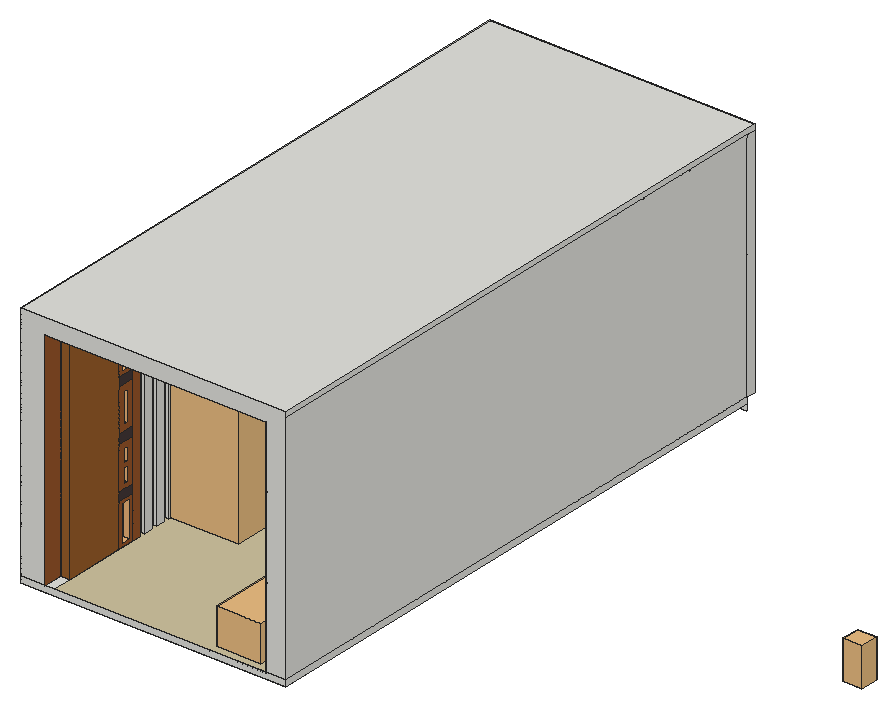
# SketchUp Ruby script. Lengths in inches.
U = 1.inch
M = Sketchup.active_model
def pt(a) = Geom::Point3d.new(a.map { |v| v * U })
def face(e, loops, mat)
  f = e.add_face(loops[0].map { |a| pt(a) })
  loops[1..].each { |l| e.add_face(l.map { |a| pt(a) }).erase! }
  f.material = f.back_material = mat if mat
  f
end
# faces: each face lists its corners as indices into pts; further lists are holes
def faces(e, pts, list, mat = nil) = list.each { |f| face(e, (f[0].is_a?(Array) ? f : [f]).map { |l| l.map { |i| pts[i] } }, mat) }
# xy, xz, yz: faces in a plane at the given z, y or x. An outline is a flat list of corners, or four numbers for a rectangle; further outlines are holes
def ring(l) = l.size == 4 ? [[l[0], l[1]], [l[2], l[1]], [l[2], l[3]], [l[0], l[3]]] : l.each_slice(2).to_a
def flat(e, list, mat, &to3) = list.each { |f| face(e, (f[0].is_a?(Array) ? f : [f]).map { |l| ring(l).map { |u, v| to3.(u, v) } }, mat) }
def xy(e, z, list, mat = nil) = flat(e, list, mat) { |x, y| [x, y, z] }
def xz(e, y, list, mat = nil) = flat(e, list, mat) { |x, z| [x, y, z] }
def yz(e, x, list, mat = nil) = flat(e, list, mat) { |y, z| [x, y, z] }
def lines(e, pts, list) = list.each { |a, b| e.add_line(pt(pts[a]), pt(pts[b])) }
# prism: a flat outline (further loops are holes) pulled along v
def prism(e, loops, v, mat = nil)
  f = face(e, loops, mat); d = Geom::Vector3d.new(v.map { |x| x * U })
  f.pushpull(f.normal.samedirection?(d) ? d.length : -d.length)
end
def box(e, o, s, mat = nil) = prism(e, [[o, [o[0] + s[0], o[1], o[2]], [o[0] + s[0], o[1] + s[1], o[2]], [o[0], o[1] + s[1], o[2]]]], [0, 0, s[2]], mat)
def at(x, y, z, deg = 0) = Geom::Transformation.translation(pt([x, y, z])) * Geom::Transformation.rotation(ORIGIN, Z_AXIS, deg.degrees)
def axes(o, x, y, z) = Geom::Transformation.new([*x, 0, *y, 0, *z, 0, *pt(o).to_a, 1])
def part(name) = M.definitions.add(name)
# library, detail: a bought-in or finely detailed component or shape, given as its bounding box
def library(name, o, s) = part(name).tap { |d| box(d.entities, o, s) }
def detail(e, o, s) = box(e.add_group.entities, o, s)
def put(e, d, t, mat = nil) = e.add_instance(d, t).tap { |i| i.material = mat if mat }
def group(e, t, mat = nil) = e.add_group.tap { |g| g.transformation = t; g.material = mat if mat }.entities
root = M.entities
M.materials.add("Generic").color = [229, 195, 154]
M.materials.add("Generic\#1").color = [68, 57, 57]
M.materials.add("Generic\#2").color = [236, 180, 120]
M.materials.add("Material__2").color = [190, 136, 85]
M.materials.add("Material__3").color = [51, 42, 44]
M.materials.add("Material__4").color = [119, 136, 107]
M.materials.add("[Carrera Marble]").color = [207, 195, 159]
M.materials.add("[Stone Brushed Khaki]").color = [221, 193, 130]
M.materials.add("[Translucent Glass Gray]").color = [128, 128, 128]
M.materials["[Translucent Glass Gray]"].alpha = 0.5
M.materials.add("[Wood Bamboo]").color = [177, 105, 43]
M.materials.add("[Wood Cherry Original]").color = [152, 86, 42]
M.materials.add("[Wood Floor Dark]").color = [153, 94, 42]
M.materials.add("[Wood Floor Light]").color = [204, 176, 127]
c1 = library("1",[-11,-10.66,0],[22,21.32,33.52])
c2 = library("Lamp+10 (1)",[0,0,0],[16.92,16.92,22.79])
c3 = library("Plant+2 (1)",[-9.13,-9.52,0],[51.76,51.77,66.88])
c4 = library("Untitled (10)",[37.47,31.74,-40.69],[40.4,38.45,82.03])
c5 = library("Plante 4",[-1.67,-6.5,0],[37.31,31.95,64.42])
c6 = library("Chair+0019",[-38.03,-22.02,-0.21],[60.63,22.85,35.01])
c7 = library("\#2",[-119.83,-119.83,113.8],[239.66,239.66,17.4])
c8 = library("\#4",[-204.92,-212.35,-236.71],[424.28,257.5,472.53])
c9 = part("\#3")
put(c9.entities,c8,axes([-0.37,309.72,0],[1.36765,0,0],[0,1.36765,0],[0,0,1.36765]),"Material__4")
c10 = library("\#1",[-174.07,-174.07,0],[348.14,348.14,140])
c11 = part("9")
put(c11.entities,c7,at(-19.94,-24.66,0),"Material__3")
put(c11.entities,c9,axes([17.67,-32.6,40.29],[0.29694,0.9549,0],[-0.21403,0.06656,0.97456],[0.9306,-0.28939,0.22414]))
put(c11.entities,c10,at(-19.94,-24.66,0),"Material__2")
c12 = library("Tlon Light 450 Ceiling 152 006",[-8.86,-8.86,-3.78],[17.72,17.72,3.56])
c13 = library("Group\#35",[0,0,0],[112.99,39.26,34.22])
c14 = library("Group\#34",[0,0,0],[22.86,20.51,35.125])
xy(root,-12,[[0,0,567.3125,1234.9375]])
xy(root,0,[[0,0,53.125,0,53.125,358.875,14.1875,358.875,14.1875,512.5,53.125,512.5,53.125,1192.5625,525.9375,1192.5625,525.9375,0,567.3125,0,567.3125,1234.9375,0,1234.9375],[53.125,0,70.75,42.6875],[53.125,42.6875,70.75,42.6875,70.75,230.375,63.625,230.375,63.625,243.8125,70.75,243.8125,70.75,262.5,63.625,262.5,63.625,275.9375,70.75,275.9375,70.75,294.625,63.625,294.625,63.625,308.0625,70.75,308.0625,70.75,326.75,63.625,326.75,63.625,340.1875,70.75,340.1875,70.75,358.875,53.125,358.875],[480.125,372.5625,525.9375,589.25],[414.96,383.4,463.77,432.21],
  [53.125,737.1875,83.6875,834.8125],[480.125,808.5625,525.9375,880.5625],[80.04,834.8125,120.17,889.86],[0,1234.9375,567.3125,1256.0625]])
xy(root,0,[[[70.75,0,525.9375,0,525.9375,372.5625,480.125,372.5625,480.125,589.25,525.9375,589.25,525.9375,808.5625,480.125,808.5625,480.125,880.5625,525.9375,880.5625,525.9375,1192.5625,53.125,1192.5625,53.125,834.8125,80.04,834.8125,80.04,1097.86,120.17,1097.86,120.17,834.8125,83.6875,834.8125,83.6875,737.1875,53.125,737.1875,53.125,512.5,14.1875,512.5,14.1875,358.875,70.75,358.875,70.75,340.1875,63.625,340.1875,63.625,326.75,70.75,326.75,70.75,308.0625,63.625,308.0625,63.625,294.625,70.75,294.625,70.75,275.9375,63.625,275.9375,63.625,262.5,70.75,262.5,70.75,243.8125,63.625,243.8125,63.625,230.375,70.75,230.375],[414.96,383.4,463.77,432.21],[427.71,817.19,465.83,860.19]]],"[Carrera Marble]")
xy(root,5.99,[[54.0625,181.68,70.75,205.7]],"Generic\#2")
xy(root,14.78,[[103.11,849.59,120.17,875.08]],"[Wood Cherry Original]")
xy(root,21.23,[[103.11,911.1,120.17,1076.63]],"[Wood Cherry Original]")
xy(root,30,[[427.71,817.19,465.83,860.19]])
xy(root,46,[[414.96,383.4,463.77,432.21]])
xy(root,83.88,[[54.0625,181.68,70.75,205.7]],"Generic\#2")
xy(root,87.33,[[103.11,911.1,120.17,1076.63]])
xy(root,93.78,[[103.11,849.59,120.17,875.08]])
xy(root,108.5625,[[80.04,834.8125,120.17,889.86],[80.04,889.86,120.17,1097.86]],"[Wood Cherry Original]")
xy(root,157.88,[[54.0625,187.75,70.75,199.62]],"Generic\#2")
xy(root,170.22,[[525.9375,0,528,372.5625]])
xy(root,172.22,[[525.9375,0,528,372.5625]])
xy(root,187.62,[[54.0625,187.75,70.75,199.62]],"Generic\#2")
xy(root,231.85,[[54.0625,187.91,70.75,199.47]],"Generic\#2")
xy(root,264,[[53.125,1192.5625,525.9375,1234.9375]])
xy(root,297.28,[[54.0625,187.91,70.75,199.47]],"Generic\#2")
xy(root,336.86,[[54.0625,183.11,70.75,204.26]],"Generic\#2")
xy(root,344.4375,[[525.9375,0,528,372.5625]])
xy(root,346.4375,[[525.9375,0,528,372.5625]])
xy(root,411.89,[[54.0625,183.11,70.75,204.26]],"Generic\#2")
xy(root,429.76,[[54.0625,186.13,70.75,201.24]],"Generic\#2")
xy(root,469.55,[[54.0625,186.13,70.75,201.24]],"Generic\#2")
xy(root,480,[[53.125,42.6875,70.75,42.6875,70.75,230.375,63.625,230.375,63.625,243.8125,70.75,243.8125,70.75,262.5,63.625,262.5,63.625,275.9375,70.75,275.9375,70.75,294.625,63.625,294.625,63.625,308.0625,70.75,308.0625,70.75,326.75,63.625,326.75,63.625,340.1875,70.75,340.1875,70.75,358.875,53.125,358.875],[480.125,372.5625,525.9375,589.25],[53.125,737.1875,83.6875,834.8125],[480.125,808.5625,525.9375,880.5625]])
xy(root,480.4375,[[[53.125,0,53.125,358.875,14.1875,358.875,14.1875,512.5,53.125,512.5,53.125,1234.9375,525.9375,1234.9375,525.9375,0],[155.5,102.38,423.56,1132.56]]],"Generic")
xy(root,502.125,[[0,1234.9375,567.3125,1256.0625]])
xy(root,502.125,[[155.5,102.38,423.56,1132.56]],"Generic")
xy(root,514.125,[[0,0,567.3125,1256.0625]])
xz(root,0,[[0,-12,567.3125,0],[0,0,53.125,0,53.125,480.4375,525.9375,480.4375,525.9375,346.4375,528,346.4375,528,344.4375,525.9375,344.4375,525.9375,172.22,528,172.22,528,170.22,525.9375,170.22,525.9375,0,567.3125,0,567.3125,514.125,0,514.125]])
xz(root,42.6875,[[53.125,0,70.75,480]],"[Wood Floor Dark]")
xz(root,102.38,[[155.5,480.4375,423.56,502.125]])
xz(root,181.68,[[54.0625,5.99,70.75,83.88]])
xz(root,183.11,[[54.0625,336.86,70.75,411.89]])
xz(root,186.13,[[54.0625,429.76,70.75,469.55]])
xz(root,187.75,[[54.0625,157.88,70.75,187.62]])
xz(root,187.91,[[54.0625,231.85,70.75,297.28]])
xz(root,188.65,[[54.0625,119.25,70.75,149.41]])
xz(root,198.45,[[54.0625,119.23,70.75,149.39]],"Generic\#2")
xz(root,199.47,[[54.0625,231.85,70.75,297.28]],"Generic\#2")
xz(root,199.62,[[54.0625,157.88,70.75,187.62]],"Generic\#2")
xz(root,201.24,[[54.0625,429.76,70.75,469.55]],"Generic\#2")
xz(root,204.26,[[54.0625,336.86,70.75,411.89]],"Generic\#2")
xz(root,205.7,[[54.0625,5.99,70.75,83.88]],"Generic\#2")
xz(root,230.375,[[63.625,0,70.75,480]])
xz(root,243.8125,[[63.625,0,70.75,480]])
xz(root,262.5,[[63.625,0,70.75,480]],"[Wood Cherry Original]")
xz(root,275.9375,[[63.625,0,70.75,480]])
xz(root,294.625,[[63.625,0,70.75,480]],"[Wood Cherry Original]")
xz(root,308.0625,[[63.625,0,70.75,480]])
xz(root,326.75,[[63.625,0,70.75,480]],"[Wood Cherry Original]")
xz(root,340.1875,[[63.625,0,70.75,480]])
xz(root,358.875,[[14.1875,0,53.125,480.4375],[14.1875,480.4375,53.125,502.125]])
xz(root,358.875,[[53.125,0,70.75,480]],"[Wood Cherry Original]")
xz(root,372.5625,[[525.9375,170.22,528,172.22],[525.9375,344.4375,528,346.4375]])
xz(root,372.5625,[[480.125,0,525.9375,480]],"[Wood Cherry Original]")
xz(root,383.4,[[414.96,0,463.77,46]])
xz(root,432.21,[[414.96,0,463.77,46]])
xz(root,512.5,[[14.1875,480.4375,53.125,502.125]])
xz(root,512.5,[[14.1875,412.1875,53.125,431.1875]],"Generic\#1")
xz(root,512.5,[[14.1875,0,53.125,412.1875]],"[Wood Floor Dark]")
xz(root,512.5,[[14.1875,431.1875,53.125,480.4375]],"[Wood Floor Light]")
xz(root,589.25,[[480.125,0,525.9375,480]],"[Wood Cherry Original]")
xz(root,737.1875,[[53.125,0,83.6875,480]],"[Wood Cherry Original]")
xz(root,808.5625,[[480.125,0,525.9375,480]],"[Wood Cherry Original]")
xz(root,817.19,[[427.71,0,465.83,30]])
xz(root,834.8125,[[53.125,0,53.125,480,83.6875,480,83.6875,108.5625,80.04,108.5625,80.04,0],[80.04,0,83.6875,108.5625]])
xz(root,834.8125,[[83.6875,0,120.17,108.5625]],"[Wood Cherry Original]")
xz(root,849.59,[[103.11,14.78,120.17,93.78]])
xz(root,860.19,[[427.71,0,465.83,30]])
xz(root,875.08,[[103.11,14.78,120.17,93.78]],"[Wood Cherry Original]")
xz(root,880.5625,[[480.125,0,525.9375,480]])
xz(root,889.86,[[80.04,0,120.17,108.5625]])
xz(root,911.1,[[103.11,21.23,120.17,87.33]])
xz(root,1076.63,[[103.11,21.23,120.17,87.33]],"[Wood Cherry Original]")
xz(root,1097.86,[[80.04,0,120.17,108.5625]])
xz(root,1132.56,[[155.5,480.4375,423.56,502.125]],"Generic")
xz(root,1192.5625,[[53.125,0,69.9375,240],[53.125,240,525.9375,264]],"[Wood Cherry Original]")
xz(root,1234.9375,[[0,-25.89,567.3125,-12],[0,-12,567.3125,0],[0,0,53.125,502.125],[53.125,0,567.3125,264],[53.125,264,525.9375,480.4375],
  [525.9375,264,567.3125,502.125],[53.125,480.4375,525.9375,502.125]])
xz(root,1256.0625,[[0,0,567.3125,502.125],[0,502.125,567.3125,514.125]])
yz(root,0,[[0,-12,1234.9375,0],[0,0,1234.9375,502.125],[1234.9375,0,1256.0625,502.125],[0,502.125,1256.0625,514.125]])
yz(root,14.1875,[[358.875,480.4375,512.5,502.125]])
yz(root,14.1875,[[358.875,0,512.5,480.4375]],"[Wood Cherry Original]")
yz(root,53.125,[[42.6875,0,358.875,480],[737.1875,0,834.8125,480],[42.6875,480,358.875,480.4375],[737.1875,480,834.8125,480.4375],[42.6875,480.4375,358.875,502.125],
  [512.5,480.4375,737.1875,502.125],[737.1875,480.4375,834.8125,502.125],[834.8125,480.4375,1234.9375,502.125]])
yz(root,53.125,[[512.5,412.1875,737.1875,431.1875]],"Generic\#1")
yz(root,53.125,[[834.8125,0,1192.5625,0,1192.5625,264,1234.9375,264,1234.9375,480.4375,834.8125,480.4375]],"[Wood Bamboo]")
yz(root,53.125,[[0,0,42.6875,480.4375]],"[Wood Cherry Original]")
yz(root,53.125,[[512.5,0,737.1875,412.1875]],"[Wood Floor Dark]")
yz(root,53.125,[[512.5,431.1875,737.1875,480.4375]],"[Wood Floor Light]")
yz(root,54.0625,[[181.68,5.99,205.7,83.88],[198.45,119.23,198.45,149.39,188.65,149.41,188.65,119.25],[187.75,157.88,199.62,187.62],[187.91,231.85,199.47,297.28],[183.11,336.86,204.26,411.89],
  [186.13,429.76,201.24,469.55]],"Generic\#2")
yz(root,63.625,[[230.375,0,243.8125,480],[262.5,0,275.9375,480],[294.625,0,308.0625,480],[326.75,0,340.1875,480]],"[Wood Cherry Original]")
yz(root,70.75,[[243.8125,0,262.5,480],[275.9375,0,294.625,480],[308.0625,0,326.75,480],[340.1875,0,358.875,480]])
yz(root,70.75,[[175.6875,89.875,211.6875,109.8125],[175.6875,199.6875,211.6875,219.625],[175.6875,309.5,211.6875,329.4375]],"Generic\#1")
yz(root,70.75,[[[175.6875,0,211.6875,89.875],[181.68,5.99,205.7,83.88]],[211.6875,0,230.375,480],[[175.6875,109.8125,211.6875,199.6875],[187.75,157.88,199.62,187.62],[198.45,119.23,188.65,119.25,188.65,149.41,198.45,149.39]],[[175.6875,219.625,211.6875,309.5],[187.91,231.85,199.47,297.28]],[[175.6875,329.4375,211.6875,419.3125],[183.11,336.86,204.26,411.89]],
  [[175.6875,419.3125,211.6875,480],[186.13,429.76,201.24,469.55]]],"[Wood Cherry Original]")
yz(root,70.75,[[42.6875,0,175.6875,480]],"[Wood Floor Dark]")
yz(root,80.04,[[834.8125,0,889.86,108.5625],[889.86,0,1097.86,108.5625]])
yz(root,83.6875,[[737.1875,0,834.8125,480]],"[Wood Cherry Original]")
yz(root,103.11,[[849.59,14.78,875.08,93.78]])
yz(root,103.11,[[911.1,21.23,1076.63,87.33]],"[Wood Cherry Original]")
yz(root,120.17,[[[834.8125,0,889.86,108.5625],[849.59,14.78,875.08,93.78]],[[889.86,0,1097.86,108.5625],[911.1,21.23,1076.63,87.33]]],"[Wood Cherry Original]")
yz(root,155.5,[[102.38,480.4375,1132.56,502.125]],"Generic")
yz(root,414.96,[[383.4,0,432.21,46]])
yz(root,423.56,[[102.38,480.4375,1132.56,502.125]],"Generic")
yz(root,427.71,[[817.19,0,860.19,30]])
yz(root,463.77,[[383.4,0,432.21,46]])
yz(root,465.83,[[817.19,0,860.19,30]])
yz(root,480.125,[[372.5625,0,589.25,480],[808.5625,0,880.5625,480]],"[Wood Cherry Original]")
yz(root,525.9375,[[372.5625,0,589.25,480],[808.5625,0,880.5625,480],[372.5625,480,589.25,480.4375],[808.5625,480,880.5625,480.4375],[372.5625,480.4375,589.25,502.125],
  [589.25,480.4375,808.5625,502.125],[808.5625,480.4375,880.5625,502.125],[880.5625,480.4375,1234.9375,502.125]])
yz(root,525.9375,[[0,0,372.5625,170.22],[0,172.22,372.5625,344.4375],[0,346.4375,372.5625,480.4375]],"[Stone Brushed Khaki]")
yz(root,525.9375,[[589.25,0,808.5625,480.4375],[880.5625,0,880.5625,480.4375,1234.9375,480.4375,1234.9375,264,1192.5625,264,1192.5625,0]],"[Wood Floor Dark]")
yz(root,528,[[0,170.22,372.5625,172.22],[0,344.4375,372.5625,346.4375]])
yz(root,567.3125,[[0,-12,1234.9375,0],[0,0,1234.9375,502.125],[1234.9375,0,1256.0625,502.125],[0,502.125,1256.0625,514.125]])
p = [[70.75,188.65,119.25],[70.75,198.45,119.23],[54.0625,198.45,119.23],[54.0625,188.65,119.25],[70.75,198.45,149.39],[70.75,188.65,149.41],
  [54.0625,188.65,149.41],[54.0625,198.45,149.39],[525.9375,1228.5625,240],[69.9375,1228.5625,240],[-38,1234.9375,0],[0,1234.9375,0],
  [525.9375,0,502.125],[525.9375,372.5625,502.125],[53.125,42.6875,502.125],[53.125,0,502.125]]
faces(root,p,[[0,1,2,3],[4,5,6,7]],"Generic\#2")
lines(root,p,[[8,9],[10,11],[12,13],[14,15]])
put(root,c1,axes([419.13,562.39,0],[0,-3.28,0],[3.28,0,0],[0,0,3.28]))
put(root,c2,axes([406.17,391.62,46],[2.83864,0,0],[0,2.83864,0],[0,0,2.83864]))
put(root,c3,axes([25.84,355.23,0],[4.47,0,0],[0,4.47,0],[0,0,4.47]))
put(root,c4,at(1745.55,-60.35,478.6))
put(root,c1,axes([419.13,483.33,0],[0,-3.28,0],[3.28,0,0],[0,0,3.28]))
put(root,c2,axes([423.5,817.19,30],[2.59659,0,0],[0,2.59659,0],[0,0,2.59659]))
put(root,c1,axes([457.15,928.65,0.07],[0,-3.28,0],[3.28,0,0],[0,0,3.28]))
put(root,c1,axes([457.15,1011.03,0.07],[0,-3.28,0],[3.28,0,0],[0,0,3.28]))
put(root,c1,axes([457.15,1093.4,0.07],[0,-3.28,0],[3.28,0,0],[0,0,3.28]))
put(root,c5,at(82.79,848.83,108.5625))
put(root,c6,at(459.57,904.68,74))
put(root,c11,axes([100.74,929.6,101.06],[0.1188,0,0],[0,0.1188,0],[0,0,0.1188]))
put(root,c11,axes([100.74,981.6,101.06],[0.1188,0,0],[0,0.1188,0],[0,0,0.1188]))
put(root,c11,axes([100.74,1033.6,101.06],[0.1188,0,0],[0,0.1188,0],[0,0,0.1188]))
put(root,c11,axes([100.74,1085.6,101.06],[0.1188,0,0],[0,0.1188,0],[0,0,0.1188]))
put(root,c12,axes([456.96,107.18,482.39],[0.75,0,0],[0,0.75,0],[0,0,0.75]))
put(root,c12,axes([456.96,107.18,481.26],[0.75,0,0],[0,0.75,0],[0,0,0.75]))
put(root,c12,axes([456.96,317.74,481.26],[0.75,0,0],[0,0.75,0],[0,0,0.75]))
put(root,c12,axes([456.96,528.3,481.26],[0.75,0,0],[0,0.75,0],[0,0,0.75]))
put(root,c12,axes([456.96,738.86,481.26],[0.75,0,0],[0,0.75,0],[0,0,0.75]))
put(root,c12,axes([456.96,949.43,481.26],[0.75,0,0],[0,0.75,0],[0,0,0.75]))
put(root,c12,axes([456.96,1159.99,481.26],[0.75,0,0],[0,0.75,0],[0,0,0.75]))
put(root,c12,axes([116.96,107.18,481.26],[0.75,0,0],[0,0.75,0],[0,0,0.75]))
put(root,c12,axes([116.96,312.11,481.26],[0.75,0,0],[0,0.75,0],[0,0,0.75]))
put(root,c12,axes([116.96,517.05,481.26],[0.75,0,0],[0,0.75,0],[0,0,0.75]))
put(root,c12,axes([116.96,721.99,481.26],[0.75,0,0],[0,0.75,0],[0,0,0.75]))
put(root,c12,axes([116.96,926.93,481.26],[0.75,0,0],[0,0.75,0],[0,0,0.75]))
put(root,c12,axes([116.96,1131.86,481.26],[0.75,0,0],[0,0.75,0],[0,0,0.75]))
g1 = group(root,at(69.9375,1192.5625,0))
xy(g1,0,[[42.6875,0,54.6875,3.1875],[97.375,0,109.375,3.1875],[152.0625,0,164.0625,3.1875],[206.75,0,218.75,3.1875],[261.4375,0,273.4375,3.1875],
  [316.125,0,328.125,3.1875],[370.8125,0,382.8125,3.1875],[425.5,0,437.5,3.1875],[0,3.1875,456,15.1875]])
xy(g1,180.875,[[0,0,42.6875,3.1875],[42.6875,0,54.6875,3.1875],[54.6875,0,97.375,3.1875],[97.375,0,109.375,3.1875],[109.375,0,152.0625,3.1875],
  [152.0625,0,164.0625,3.1875],[164.0625,0,206.75,3.1875],[206.75,0,218.75,3.1875],[218.75,0,261.4375,3.1875],[261.4375,0,273.4375,3.1875],
  [273.4375,0,316.125,3.1875],[316.125,0,328.125,3.1875],[328.125,0,370.8125,3.1875],[370.8125,0,382.8125,3.1875],[382.8125,0,425.5,3.1875],
  [425.5,0,437.5,3.1875],[437.5,0,456,3.1875]])
xy(g1,192.875,[[0,0,42.6875,3.1875],[42.6875,0,54.6875,3.1875],[54.6875,0,97.375,3.1875],[97.375,0,109.375,3.1875],[109.375,0,152.0625,3.1875],
  [152.0625,0,164.0625,3.1875],[164.0625,0,206.75,3.1875],[206.75,0,218.75,3.1875],[218.75,0,261.4375,3.1875],[261.4375,0,273.4375,3.1875],
  [273.4375,0,316.125,3.1875],[316.125,0,328.125,3.1875],[328.125,0,370.8125,3.1875],[370.8125,0,382.8125,3.1875],[382.8125,0,425.5,3.1875],
  [425.5,0,437.5,3.1875],[437.5,0,456,3.1875]])
xy(g1,240,[[42.6875,0,54.6875,3.1875],[97.375,0,109.375,3.1875],[152.0625,0,164.0625,3.1875],[206.75,0,218.75,3.1875],[261.4375,0,273.4375,3.1875],
  [316.125,0,328.125,3.1875],[370.8125,0,382.8125,3.1875],[425.5,0,437.5,3.1875],[0,3.1875,456,15.1875]])
xz(g1,0,[[42.6875,0,54.6875,180.875],[97.375,0,109.375,180.875],[152.0625,0,164.0625,180.875],[206.75,0,218.75,180.875],[261.4375,0,273.4375,180.875],
  [316.125,0,328.125,180.875],[370.8125,0,382.8125,180.875],[425.5,0,437.5,180.875],[0,180.875,42.6875,192.875],[42.6875,180.875,54.6875,192.875],
  [54.6875,180.875,97.375,192.875],[97.375,180.875,109.375,192.875],[109.375,180.875,152.0625,192.875],[152.0625,180.875,164.0625,192.875],[164.0625,180.875,206.75,192.875],
  [206.75,180.875,218.75,192.875],[218.75,180.875,261.4375,192.875],[261.4375,180.875,273.4375,192.875],[273.4375,180.875,316.125,192.875],[316.125,180.875,328.125,192.875],
  [328.125,180.875,370.8125,192.875],[370.8125,180.875,382.8125,192.875],[382.8125,180.875,425.5,192.875],[425.5,180.875,437.5,192.875],[437.5,180.875,456,192.875],
  [42.6875,192.875,54.6875,240],[97.375,192.875,109.375,240],[152.0625,192.875,164.0625,240],[206.75,192.875,218.75,240],[261.4375,192.875,273.4375,240],
  [316.125,192.875,328.125,240],[370.8125,192.875,382.8125,240],[425.5,192.875,437.5,240]])
xz(g1,3.1875,[[42.6875,0,54.6875,180.875],[97.375,0,109.375,180.875],[152.0625,0,164.0625,180.875],[206.75,0,218.75,180.875],[261.4375,0,273.4375,180.875],
  [316.125,0,328.125,180.875],[370.8125,0,382.8125,180.875],[425.5,0,437.5,180.875],[42.6875,192.875,54.6875,240],[97.375,192.875,109.375,240],
  [152.0625,192.875,164.0625,240],[206.75,192.875,218.75,240],[261.4375,192.875,273.4375,240],[316.125,192.875,328.125,240],[370.8125,192.875,382.8125,240],
  [425.5,192.875,437.5,240]])
xz(g1,3.1875,[[0,0,42.6875,180.875],[54.6875,0,97.375,180.875],[109.375,0,152.0625,180.875],[164.0625,0,206.75,180.875],[218.75,0,261.4375,180.875],
  [273.4375,0,316.125,180.875],[328.125,0,370.8125,180.875],[382.8125,0,425.5,180.875],[437.5,0,456,180.875],[0,192.875,42.6875,240],
  [54.6875,192.875,97.375,240],[109.375,192.875,152.0625,240],[164.0625,192.875,206.75,240],[218.75,192.875,261.4375,240],[273.4375,192.875,316.125,240],
  [328.125,192.875,370.8125,240],[382.8125,192.875,425.5,240],[437.5,192.875,456,240]],"[Translucent Glass Gray]")
yz(g1,0,[[3.1875,0,3.1875,180.875,0,180.875,0,192.875,15.1875,192.875,15.1875,0],[3.1875,192.875,15.1875,240]])
yz(g1,42.6875,[[0,0,3.1875,180.875],[0,192.875,3.1875,240]])
yz(g1,54.6875,[[0,0,3.1875,180.875],[0,192.875,3.1875,240]])
yz(g1,97.375,[[0,0,3.1875,180.875],[0,192.875,3.1875,240]])
yz(g1,109.375,[[0,0,3.1875,180.875],[0,192.875,3.1875,240]])
yz(g1,152.0625,[[0,0,3.1875,180.875],[0,192.875,3.1875,240]])
yz(g1,164.0625,[[0,0,3.1875,180.875],[0,192.875,3.1875,240]])
yz(g1,206.75,[[0,0,3.1875,180.875],[0,192.875,3.1875,240]])
yz(g1,218.75,[[0,0,3.1875,180.875],[0,192.875,3.1875,240]])
yz(g1,261.4375,[[0,0,3.1875,180.875],[0,192.875,3.1875,240]])
yz(g1,273.4375,[[0,0,3.1875,180.875],[0,192.875,3.1875,240]])
yz(g1,316.125,[[0,0,3.1875,180.875],[0,192.875,3.1875,240]])
yz(g1,328.125,[[0,0,3.1875,180.875],[0,192.875,3.1875,240]])
yz(g1,370.8125,[[0,0,3.1875,180.875],[0,192.875,3.1875,240]])
yz(g1,382.8125,[[0,0,3.1875,180.875],[0,192.875,3.1875,240]])
yz(g1,425.5,[[0,0,3.1875,180.875],[0,192.875,3.1875,240]])
yz(g1,437.5,[[0,0,3.1875,180.875],[0,192.875,3.1875,240]])
yz(g1,456,[[3.1875,0,15.1875,0,15.1875,192.875,0,192.875,0,180.875,3.1875,180.875],[3.1875,192.875,15.1875,240]])
g2 = group(root,at(69.9375,1209.4375,264))
xy(g2,0,[[57.375,0,69.375,4.8125],[126.75,0,138.75,4.8125],[196.125,0,208.125,4.8125],[265.5,0,277.5,4.8125],[334.875,0,346.875,4.8125],
  [404.25,0,416.25,4.8125]])
xy(g2,216,[[57.375,0,69.375,4.8125],[126.75,0,138.75,4.8125],[196.125,0,208.125,4.8125],[265.5,0,277.5,4.8125],[334.875,0,346.875,4.8125],
  [404.25,0,416.25,4.8125],[0,4.8125,456,16.8125]])
xz(g2,0,[[57.375,0,69.375,216],[126.75,0,138.75,216],[196.125,0,208.125,216],[265.5,0,277.5,216],[334.875,0,346.875,216],
  [404.25,0,416.25,216]])
xz(g2,4.8125,[[57.375,0,69.375,216],[126.75,0,138.75,216],[196.125,0,208.125,216],[265.5,0,277.5,216],[334.875,0,346.875,216],
  [404.25,0,416.25,216]])
xz(g2,4.8125,[[69.375,0,126.75,216],[138.75,0,196.125,216],[208.125,0,265.5,216],[277.5,0,334.875,216],[346.875,0,404.25,216],
  [416.25,0,456,216]],"[Translucent Glass Gray]")
xz(g2,16.8125,[[0,0,456,216]],"[Translucent Glass Gray]")
yz(g2,57.375,[[0,0,4.8125,216]])
yz(g2,69.375,[[0,0,4.8125,216]])
yz(g2,126.75,[[0,0,4.8125,216]])
yz(g2,138.75,[[0,0,4.8125,216]])
yz(g2,196.125,[[0,0,4.8125,216]])
yz(g2,208.125,[[0,0,4.8125,216]])
yz(g2,265.5,[[0,0,4.8125,216]])
yz(g2,277.5,[[0,0,4.8125,216]])
yz(g2,334.875,[[0,0,4.8125,216]])
yz(g2,346.875,[[0,0,4.8125,216]])
yz(g2,404.25,[[0,0,4.8125,216]])
yz(g2,416.25,[[0,0,4.8125,216]])
yz(g2,456,[[4.8125,0,16.8125,216]])
put(root,c13,axes([414.17,371.48,7.61],[0,-1.5834,0],[2.39743,0,0],[0,0,2.24843]))
put(root,c14,axes([159.48,1089.6,401.41],[4.61619,0,0],[0,4.4281,0],[0,0,2.8672]))
put(root,c13,axes([414.17,186.91,7.61],[0,-1.5834,0],[2.39743,0,0],[0,0,2.24843]))
put(root,c13,axes([444.27,773.98,7.61],[0,-1.5834,0],[1.6309,0,0],[0,0,2.24843]))
put(root,c14,axes([195.1,642.01,401.41],[4.61619,0,0],[0,4.4281,0],[0,0,2.8672]))
put(root,c14,axes([230.72,194.42,401.41],[4.61619,0,0],[0,4.4281,0],[0,0,2.8672]))
